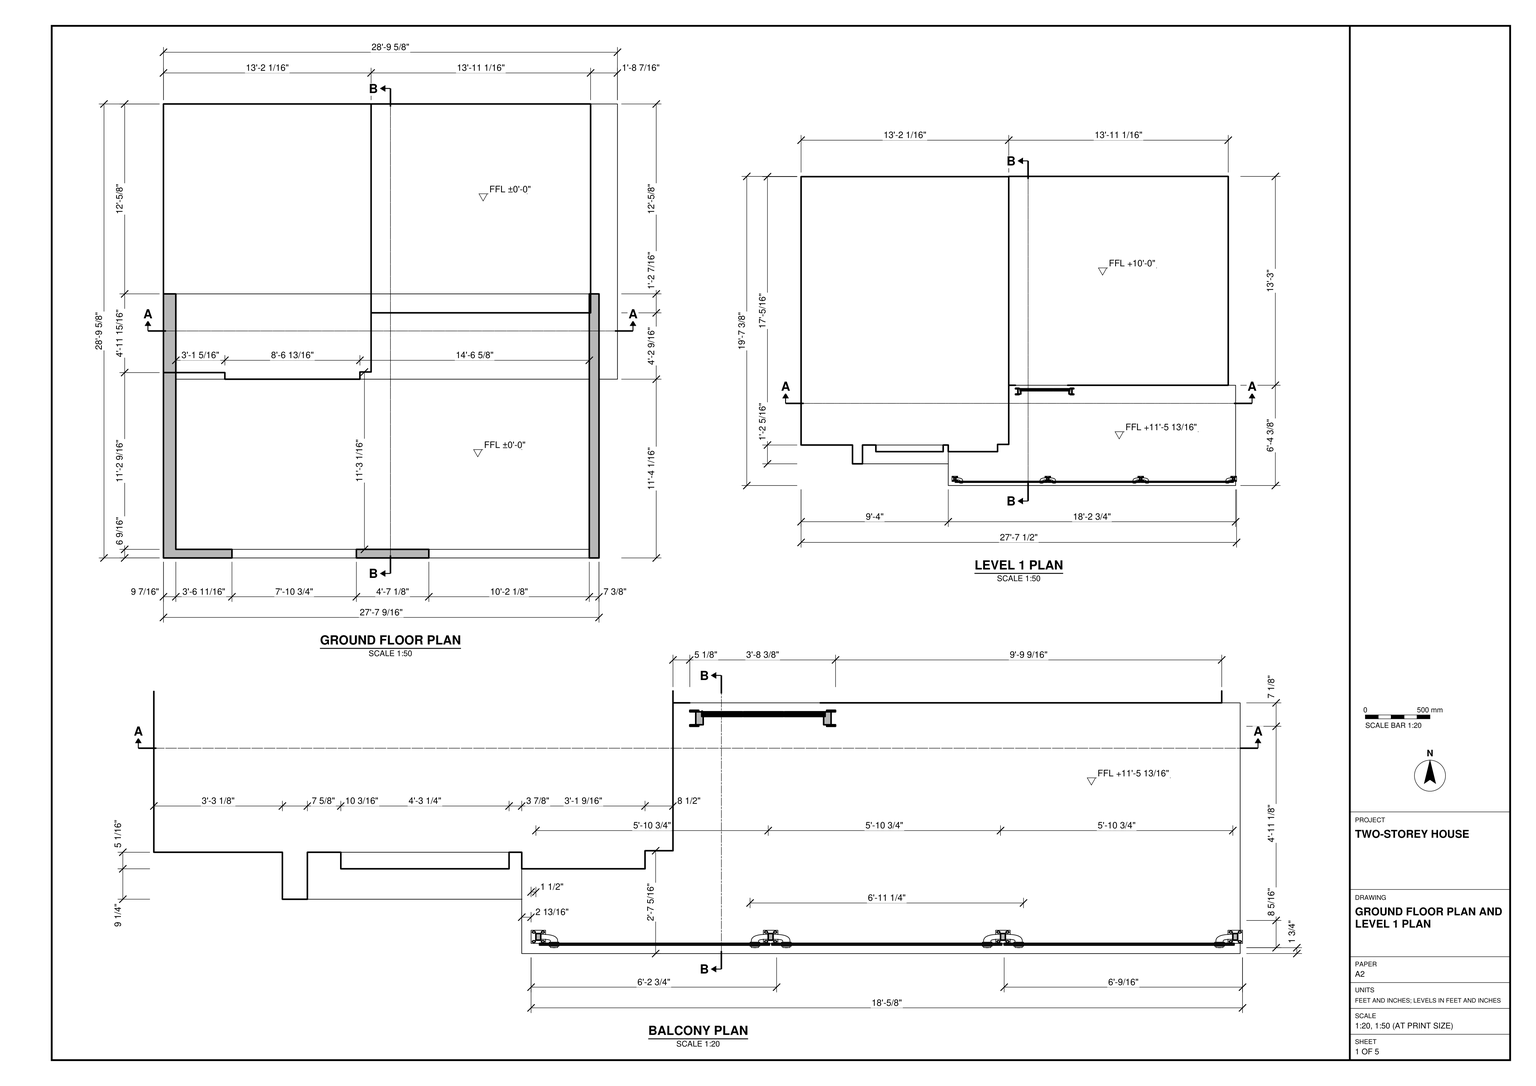
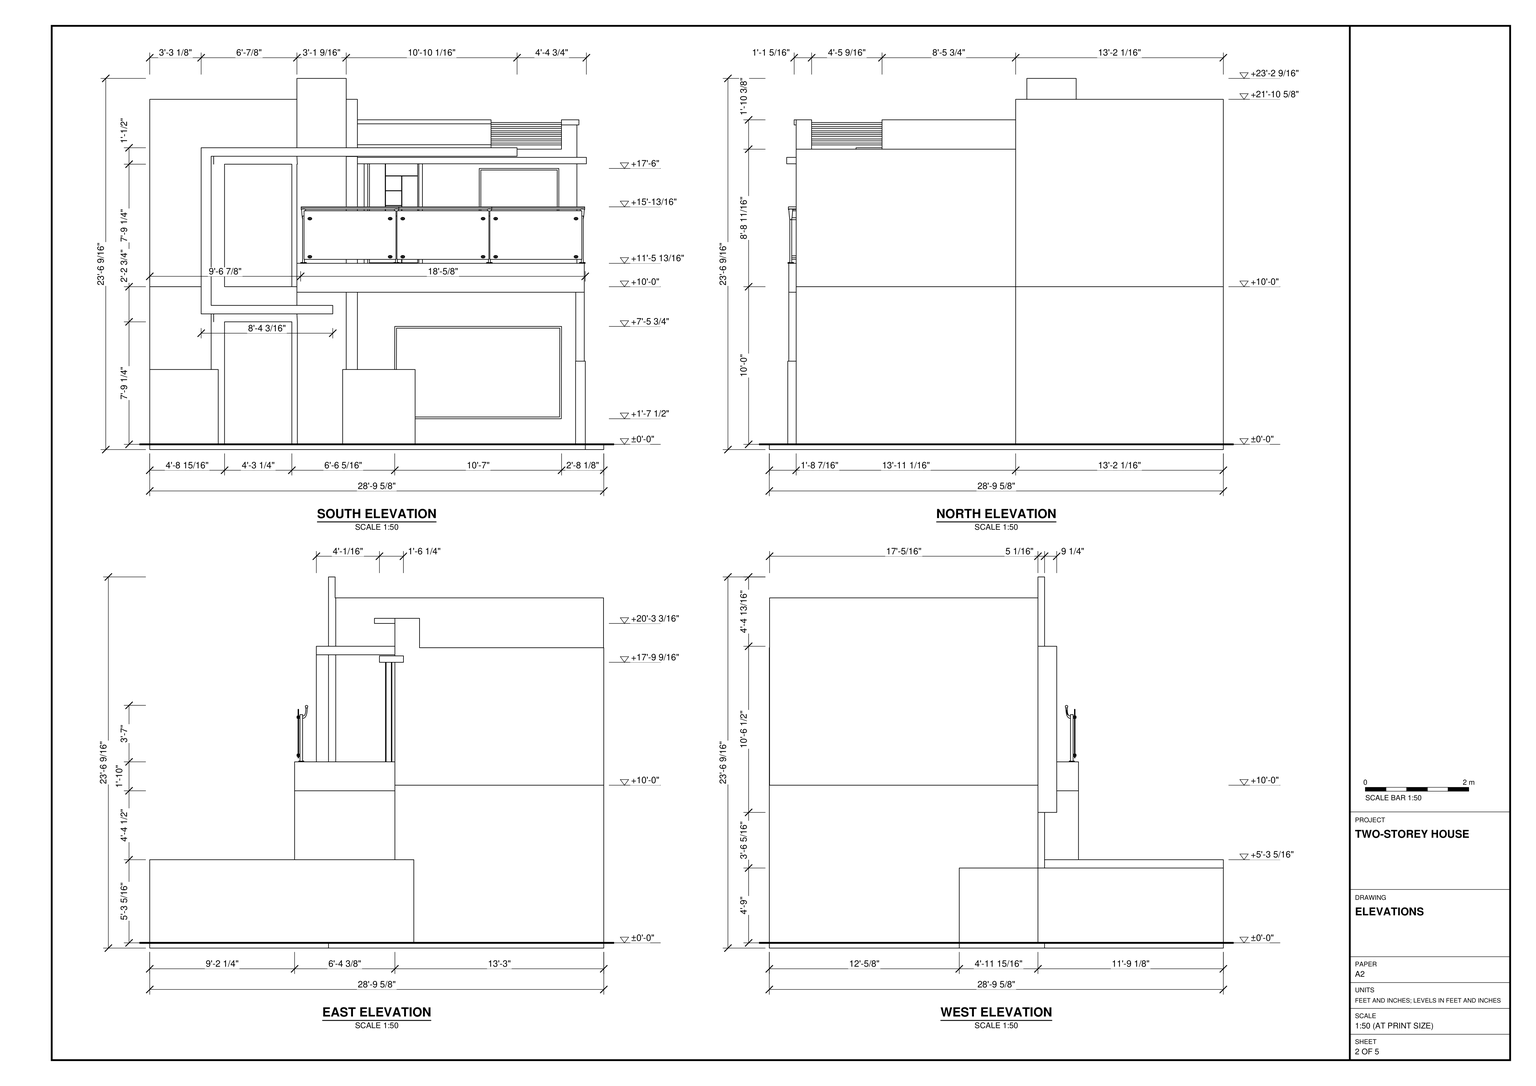
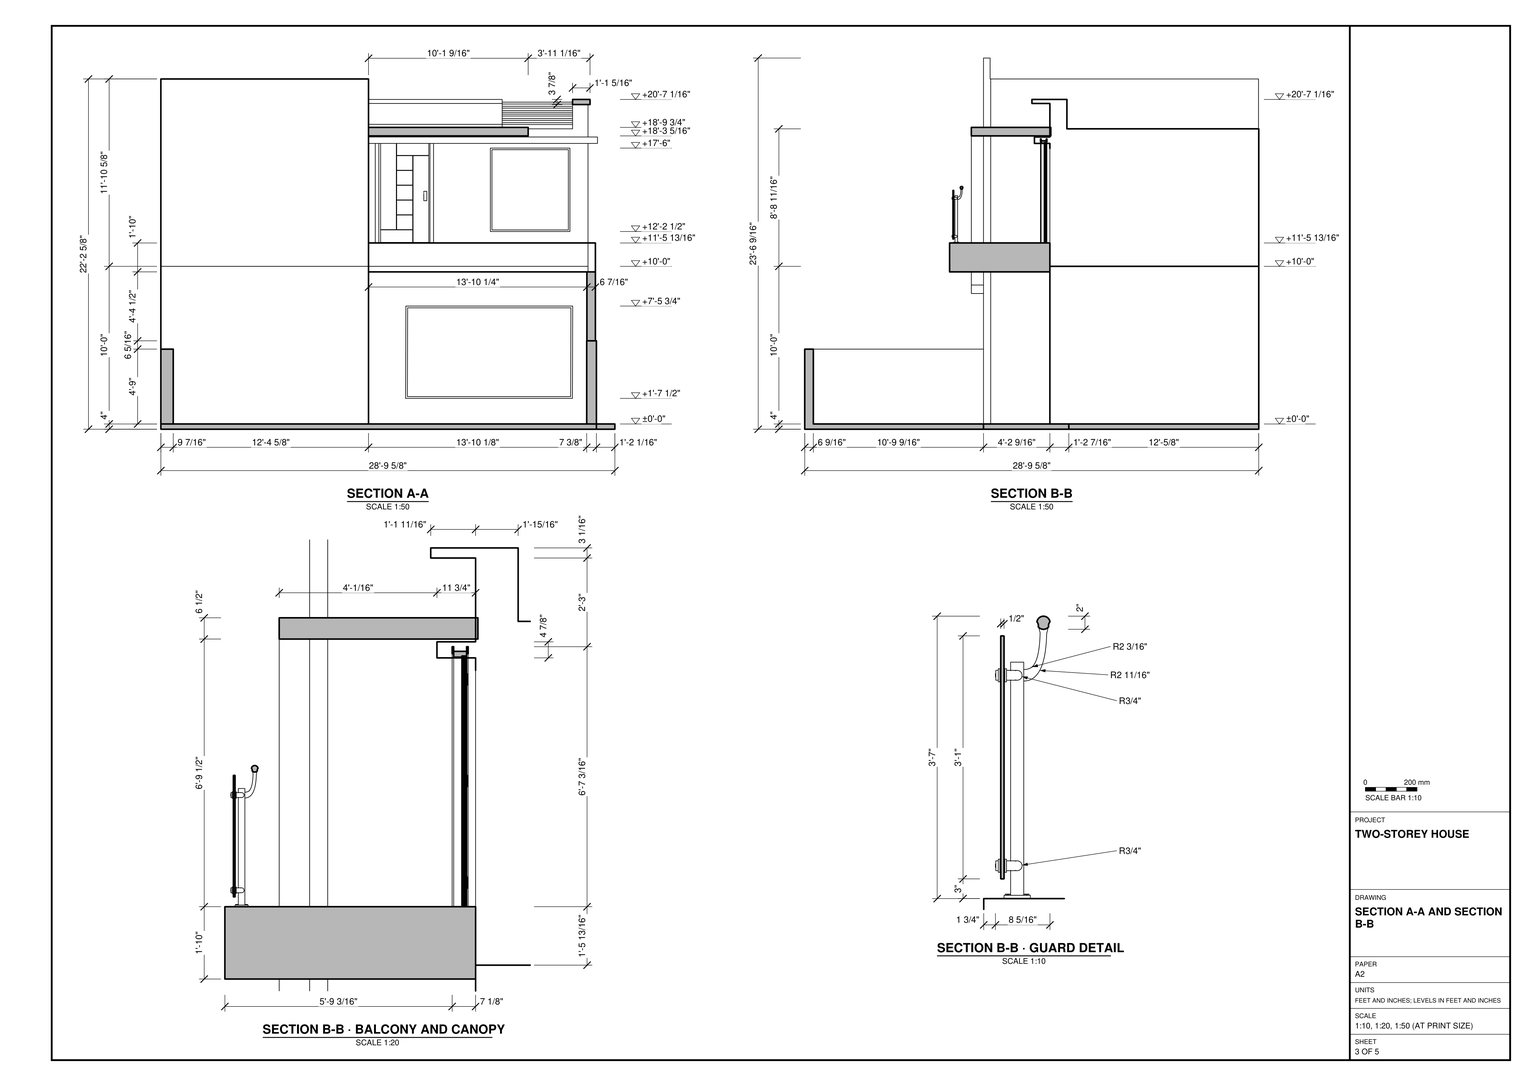
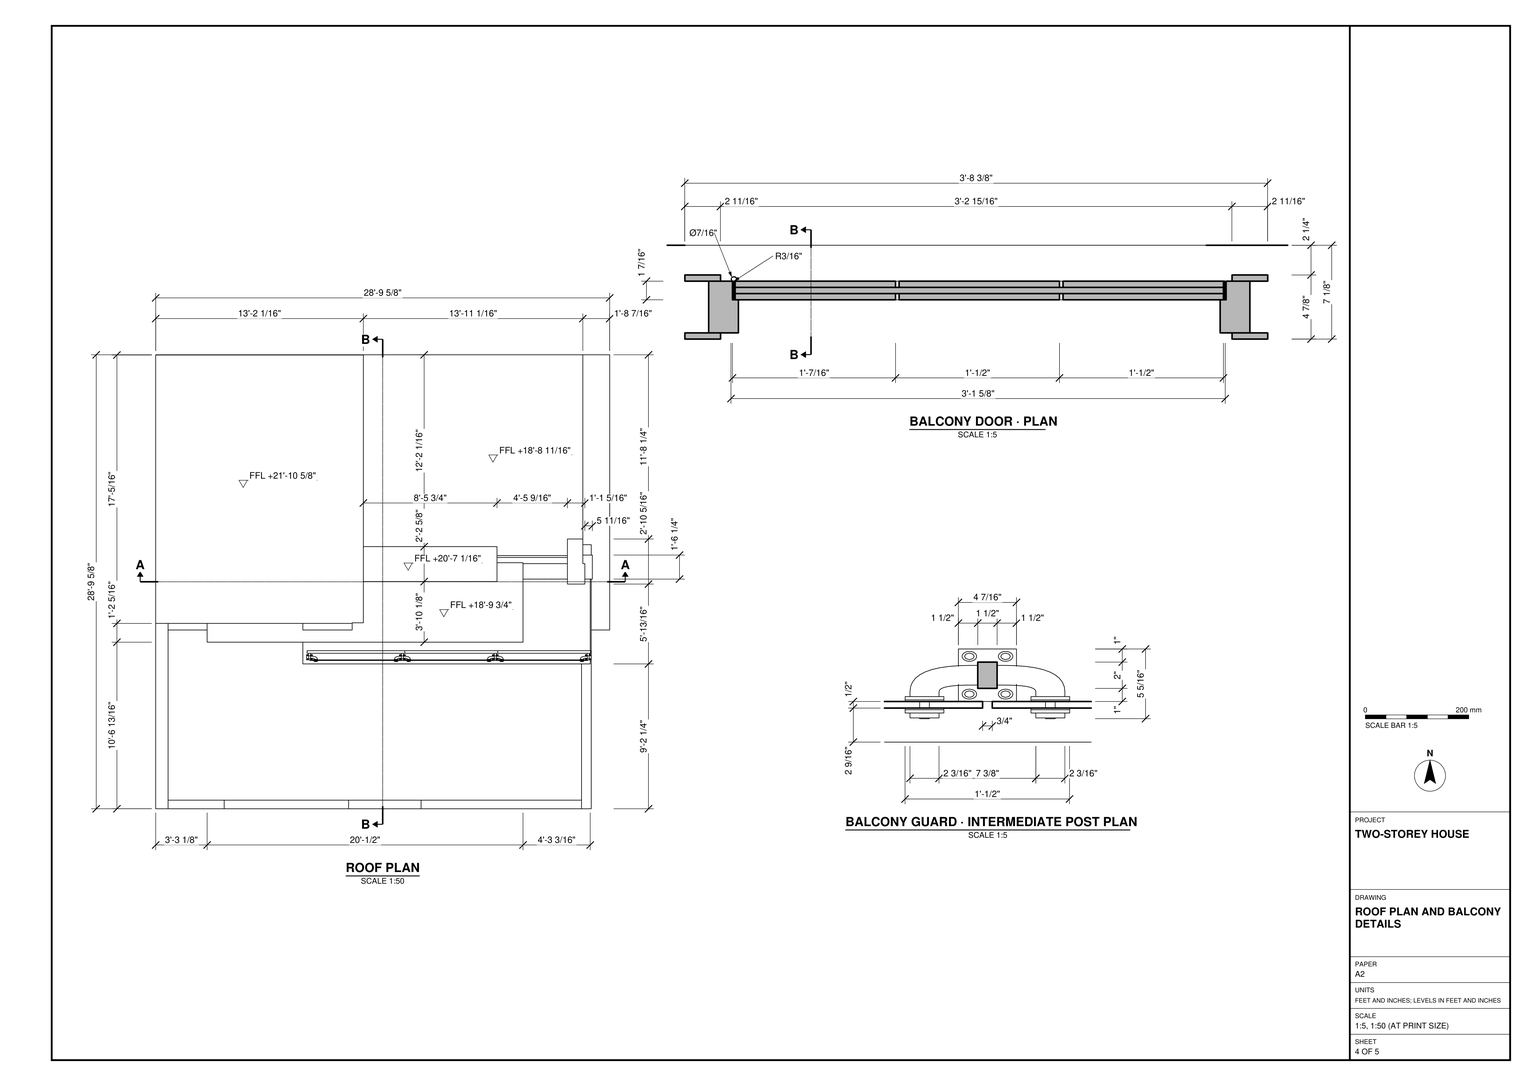
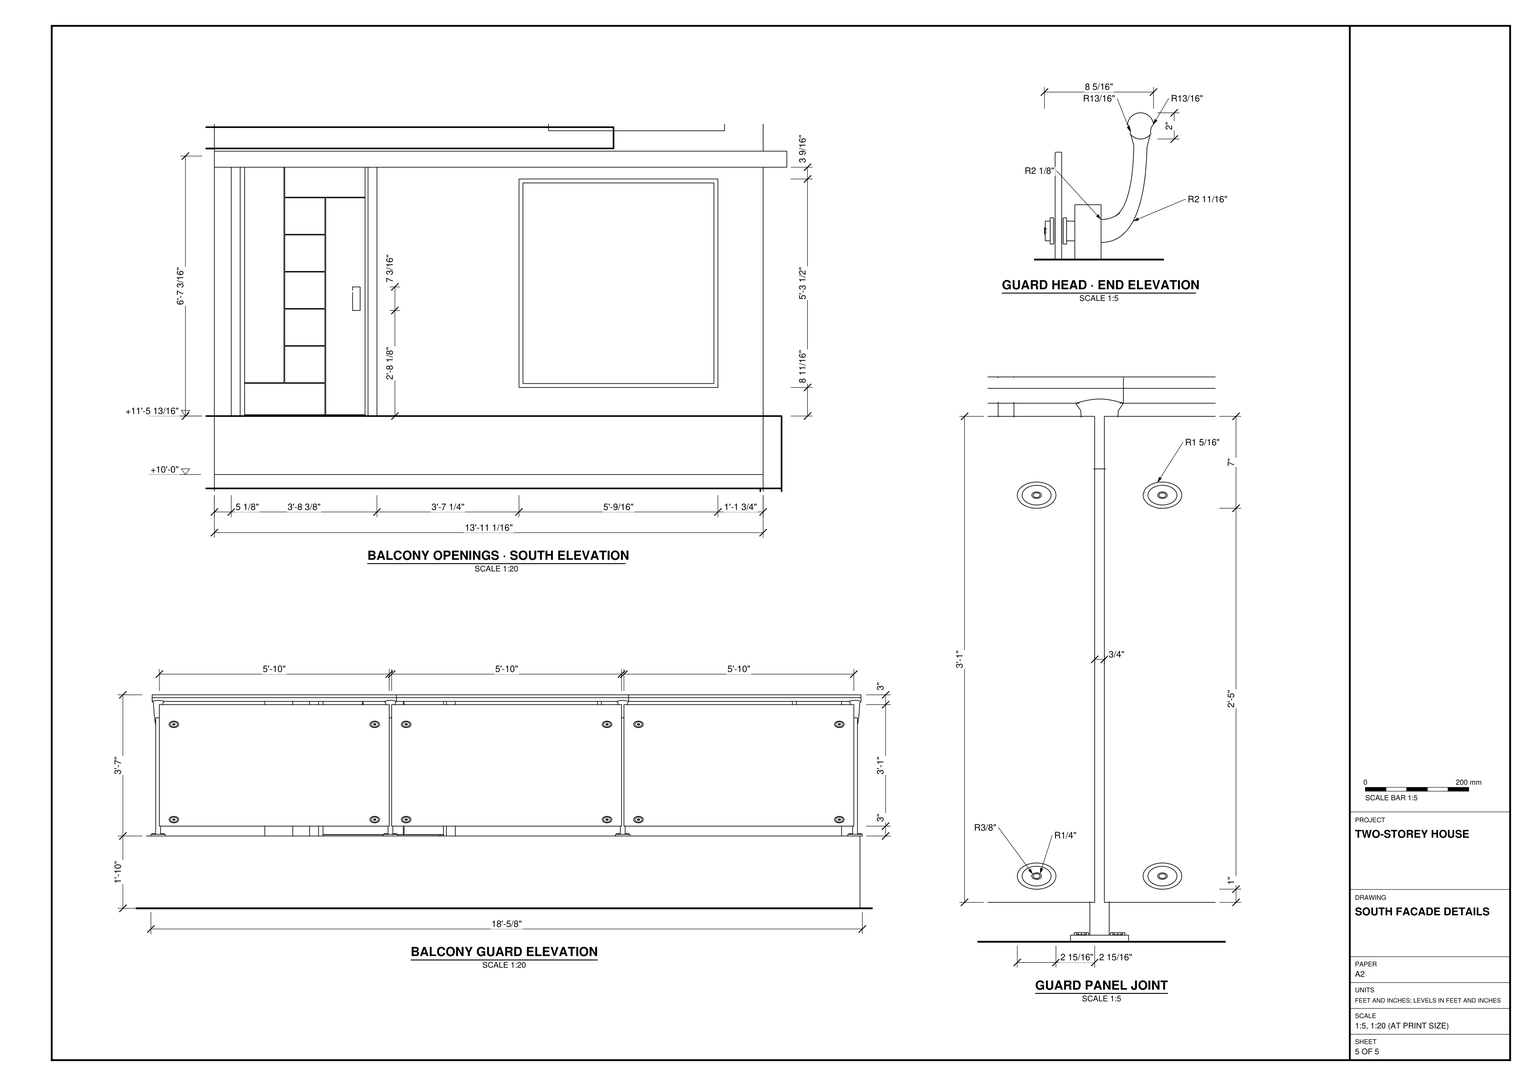
Build the two-storey house in SketchUp from task_files/diagram_01.pdf. Work in feet and inches. The model measures 28'-9 5/8" east to west, 28'-9 5/8" north to south and 23'-6 9/16" overall in height. Set the ground floor at ±0'-0" and the upper floor at +10'-0". The balcony surface is higher than the upper floor, at +11'-5 13/16".

Start with the square base slab and use the plans to position the taller west block and the recessed east bay. Model the walls at their drawn thicknesses, including the low side walls and the short wall sections that leave gaps along the south edge. Follow the elevations for the flat roofs, stepped parapets and projecting frame on the south face. Set the broad ground-floor window below the balcony and place the upper door and window behind it. Use the balcony plan for the slab outline and the sections for the canopy projection and guard construction. Show the glass panels, posts, panel fixings and offset handrail.

Keep walls, slabs and roofs in separate groups or components, and do the same for each furniture or joinery piece shown. Use components for repeated parts such as railing posts. Any decor or loose items shown may be suitable library components. Save one SketchUp model as output_files/two_storey_house_with_a_raised_front_balcony.skp.

# SketchUp Ruby script. Lengths in inches.
U = 1.inch
M = Sketchup.active_model
def pt(a) = Geom::Point3d.new(a.map { |v| v * U })
def face(e, loops, mat)
  f = e.add_face(loops[0].map { |a| pt(a) })
  loops[1..].each { |l| e.add_face(l.map { |a| pt(a) }).erase! }
  f.material = f.back_material = mat if mat
  f
end
# faces: each face lists its corners as indices into pts; further lists are holes
def faces(e, pts, list, mat = nil) = list.each { |f| face(e, (f[0].is_a?(Array) ? f : [f]).map { |l| l.map { |i| pts[i] } }, mat) }
# xy, xz, yz: faces in a plane at the given z, y or x. An outline is a flat list of corners, or four numbers for a rectangle; further outlines are holes
def ring(l) = l.size == 4 ? [[l[0], l[1]], [l[2], l[1]], [l[2], l[3]], [l[0], l[3]]] : l.each_slice(2).to_a
def flat(e, list, mat, &to3) = list.each { |f| face(e, (f[0].is_a?(Array) ? f : [f]).map { |l| ring(l).map { |u, v| to3.(u, v) } }, mat) }
def xy(e, z, list, mat = nil) = flat(e, list, mat) { |x, y| [x, y, z] }
def xz(e, y, list, mat = nil) = flat(e, list, mat) { |x, z| [x, y, z] }
def yz(e, x, list, mat = nil) = flat(e, list, mat) { |y, z| [x, y, z] }
def lines(e, pts, list) = list.each { |a, b| e.add_line(pt(pts[a]), pt(pts[b])) }
# prism: a flat outline (further loops are holes) pulled along v
def prism(e, loops, v, mat = nil)
  f = face(e, loops, mat); d = Geom::Vector3d.new(v.map { |x| x * U })
  f.pushpull(f.normal.samedirection?(d) ? d.length : -d.length)
end
def box(e, o, s, mat = nil) = prism(e, [[o, [o[0] + s[0], o[1], o[2]], [o[0] + s[0], o[1] + s[1], o[2]], [o[0], o[1] + s[1], o[2]]]], [0, 0, s[2]], mat)
def at(x, y, z, deg = 0) = Geom::Transformation.translation(pt([x, y, z])) * Geom::Transformation.rotation(ORIGIN, Z_AXIS, deg.degrees)
def axes(o, x, y, z) = Geom::Transformation.new([*x, 0, *y, 0, *z, 0, *pt(o).to_a, 1])
def part(name) = M.definitions.add(name)
# library, detail: a bought-in or finely detailed component or shape, given as its bounding box
def library(name, o, s) = part(name).tap { |d| box(d.entities, o, s) }
def detail(e, o, s) = box(e.add_group.entities, o, s)
def put(e, d, t, mat = nil) = e.add_instance(d, t).tap { |i| i.material = mat if mat }
def group(e, t, mat = nil) = e.add_group.tap { |g| g.transformation = t; g.material = mat if mat }.entities
root = M.entities
M.materials.add("B07_Copper_Blaze").color = [153, 35, 0]
M.materials.add("B08_Burnt_Sienna").color = [102, 25, 0]
M.materials.add("C02_Golden_Beige").color = [255, 205, 155]
M.materials.add("C07_Caramel_Shine").color = [153, 76, 0]
M.materials.add("D04_Dandelion_Burst").color = [255, 204, 50]
M.materials.add("E06_Meadow_Fresh").color = [204, 204, 0]
M.materials.add("Generic").color = [255, 255, 255]
M.materials.add("Glass_Basic_01").color = [161, 173, 186]
M.materials["Glass_Basic_01"].alpha = 0.25
M.materials.add("Glass_Safety_01").color = [204, 235, 244]
M.materials["Glass_Safety_01"].alpha = 0.25
M.materials.add("Glass_Safety_1").color = [204, 235, 244]
M.materials["Glass_Safety_1"].alpha = 0.25
M.materials.add("Grid_60x30_2K").color = [253, 253, 253]
M.materials.add("Marble_01_1K").color = [230, 221, 211]
M.materials.add("Marble_06_1K").color = [165, 150, 147]
M.materials.add("Plank_Floor_1K").color = [252, 252, 252]
c1 = library("CP-00619 (91x220)",[-1.57,-0.47,0],[38.58,7.14,88.1875])
c2 = library("GlassRailing",[-49.5,-2.3125,0],[147,8.3,43])
box(root,[324.32,110.28,67.3],[6.47,76.34,52.47])
xy(root,0,[[324.21,0,325.17,186.625]])
xy(root,124,[[158.08,186.625,325.17,345.64]])
xy(root,217.57,[[158.08,174.86,158.08,186.625,325.17,186.625,325.17,193.14,332.39,193.14,332.39,174.86]],"D04_Dandelion_Burst")
xy(root,222.47,[[158.08,174.86,332.39,174.86,332.39,193.14,325.17,193.14,325.17,186.625,158.08,186.625]],"D04_Dandelion_Burst")
xy(root,228.68,[[259.82,186.625,313.41,186.625,313.41,205.38,325.17,205.38,325.17,345.64,158.08,345.64,158.08,199.59,259.82,199.59]])
xy(root,235.04,[[259.82,191.32,313.41,192.75]])
xy(root,236.44,[[259.82,191.32,313.41,192.75]])
xy(root,238.48,[[259.63,191.32,313.41,192.75]])
xy(root,239.88,[[259.63,191.32,313.41,192.75]])
xy(root,241.24,[[259.59,191.32,313.41,192.75]])
xy(root,242.64,[[259.59,191.32,313.41,192.75]])
xy(root,244.45,[[259.82,191.32,313.41,192.75]])
xy(root,245.85,[[259.82,191.32,313.41,192.75]])
xy(root,247.17,[[313.41,171.07,326.7,186.625]])
xy(root,247.59,[[259.34,191.32,313.41,192.75]])
xy(root,247.98,[[158.08,172.97,259.82,186.625]],"Plank_Floor_1K")
xy(root,248.99,[[259.34,191.32,313.41,192.75]])
xy(root,251.05,[[313.41,171.07,326.7,171.07,326.7,186.625,325.17,186.625,325.17,205.38,313.41,205.38],[158.08,172.97,259.82,199.59]])
xz(root,171.07,[[313.41,247.17,326.7,251.05]])
xz(root,172.97,[[158.08,247.98,259.82,251.05]],"C02_Golden_Beige")
xz(root,174.86,[[158.08,217.57,332.39,222.47]],"D04_Dandelion_Burst")
xz(root,186.625,[[[158.08,124,325.17,217.57],[250.84,150.5,311.4,214],[163.21,141.8,202.89,213.79]],[158.08,222.47,325.17,222.47,325.17,247.17,313.41,247.17,313.41,228.68,259.82,228.68,259.82,232.1,158.08,232.1],[325.17,247.17,326.7,251.05]])
xz(root,186.625,[[[250.84,150.5,311.4,214],[252.04,151.71,310.2,212.8]]],"E06_Meadow_Fresh")
xz(root,186.625,[[252.04,151.71,310.2,212.8]],"Glass_Safety_1")
xz(root,186.625,[[158.08,232.1,259.82,247.98]],"Plank_Floor_1K")
xz(root,191.32,[[259.82,231.95,313.41,233.35],[259.82,235.04,313.41,236.44],[259.63,238.48,313.41,239.88],[259.59,241.24,313.41,242.64],[259.82,244.45,313.41,245.85],
  [259.34,247.59,313.41,248.99]])
xz(root,192.75,[[259.82,235.04,313.41,236.44],[259.63,238.48,313.41,239.88],[259.59,241.24,313.41,242.64],[259.82,244.45,313.41,245.85],[259.34,247.59,313.41,248.99]])
xz(root,193.14,[[325.17,217.57,332.39,222.47]])
xz(root,199.59,[[158.08,228.68,259.82,251.05]])
xz(root,205.38,[[313.41,228.68,325.17,251.05]])
xz(root,345.64,[[158.08,124,325.17,228.68]])
yz(root,158.08,[[186.625,124,186.625,217.57,174.86,217.57,174.86,222.47,186.625,222.47,186.625,247.98,172.97,247.98,172.97,251.05,199.59,251.05,199.59,228.68,345.64,228.68,345.64,124]])
yz(root,259.34,[[191.32,247.59,192.75,248.99]])
yz(root,259.59,[[191.32,241.24,192.75,242.64]])
yz(root,259.63,[[191.32,238.48,192.75,239.88]])
yz(root,259.82,[[[186.625,228.68,199.59,228.68,199.59,251.05,172.97,251.05,172.97,247.98,186.625,247.98],[191.32,235.04,192.75,236.44],[191.32,244.45,192.75,245.85]]])
yz(root,313.41,[[[186.625,228.68,186.625,247.17,171.07,247.17,171.07,251.05,205.38,251.05,205.38,228.68],[191.32,247.59,192.75,248.99],[191.32,244.45,192.75,245.85],[191.32,241.24,192.75,242.64],[191.32,238.48,192.75,239.88],[191.32,235.04,192.75,236.44]]])
yz(root,325.17,[[186.625,124,345.64,124,345.64,228.68,205.38,228.68,205.38,251.05,186.625,251.05,186.625,222.47,193.14,222.47,193.14,217.57,186.625,217.57]])
yz(root,326.7,[[171.07,247.17,186.625,251.05]])
yz(root,332.39,[[174.86,217.57,193.14,222.47]],"D04_Dandelion_Burst")
p = [[313.41,192.75,233.35],[259.82,192.75,233.35]]
lines(root,p,[[0,1]])
put(root,c1,axes([165.02,179.96,141.8],[1.15,0,0],[0,1,0],[0,0,0.89784]))
put(root,c2,axes([187.8125,114.37,141.8],[1.47371,0,0],[0,1,0],[0,0,1]))
g1 = group(root,at(24.45,136.09,0))
box(g1,[-24.45,0,0],[345.62,209.54,4])
g2 = group(root,at(0,126.82,4))
xy(g2,0,[[46.75,9.27,46.75,14.31,0,14.31,0,218.8125,158.08,218.8125,158.08,14.77,149.57,14.77,149.57,9.27],[158.08,59.81,325.17,218.8125]])
xy(g2,99.3,[[46.75,0,48.67,9.27],[48.67,0,49.05,9.27],[49.05,0,139.32,9.27]])
xy(g2,99.3,[[39.14,0,46.75,14.31]],"Plank_Floor_1K")
xy(g2,105.78,[[46.75,0,139.32,0,139.32,9.27,112.03,9.27,112.03,14.31,46.75,14.31]])
xy(g2,115.77,[[112.03,-16.54,112.03,9.27,149.57,9.27,149.57,14.77,158.08,14.77,158.08,59.81,330.79,59.81,330.79,-16.54]],"Marble_06_1K")
xy(g2,120,[[56.9375,9.27,108.17,14.31],[158.08,59.81,325.17,218.8125],[0,218.62,158.08,218.8125]])
xy(g2,137.8,[[112.03,-16.54,330.79,-16.54,330.79,59.81,158.08,59.81,158.08,14.77,149.57,14.77,149.57,9.27,112.03,9.27]],"Generic")
xy(g2,213.26,[[56.9375,9.27,108.17,14.31],[112.03,9.27,112.36,14.31]],"C07_Caramel_Shine")
xy(g2,219.3,[[46.75,0,48.67,14.31],[48.67,0,49.05,14.31],[49.05,0,49.05,14.31,112.03,14.31,112.03,9.27,149.57,9.27,149.57,14.77,158.08,14.77,158.08,60.51,279.62,60.51,279.62,0]])
xy(g2,225.78,[[39.14,0,279.62,0,279.62,60.51,158.08,60.51,158.08,14.77,149.57,14.77,149.57,9.27,112.03,9.27,112.03,14.31,39.14,14.31]],"Plank_Floor_1K")
xy(g2,262.64,[[0,14.31,149.57,14.31,149.57,14.77,158.08,14.77,158.08,218.62,0,218.62]])
xy(g2,278.58,[[112.03,9.27,149.57,14.31]])
xz(g2,-16.54,[[112.03,115.77,330.79,137.8]],"Generic")
xz(g2,0,[[39.14,99.3,139.32,99.3,139.32,105.78,46.75,105.78,46.75,219.3,279.62,219.3,279.62,225.78,39.14,225.78]],"Plank_Floor_1K")
xz(g2,9.27,[[46.75,0,56.9375,0,56.9375,93.26,108.17,93.26,108.17,0,112.36,0,112.36,93.26,112.03,99.3,46.75,99.3]],"B07_Copper_Blaze")
xz(g2,9.27,[[56.9375,0,108.17,93.26],[56.9375,120,108.17,213.26]],"Glass_Basic_01")
xz(g2,9.27,[[112.36,0,149.57,0,149.57,115.77,112.03,115.77,112.03,105.78,139.32,105.78,139.32,99.3,112.03,99.3,112.36,93.26],[112.03,137.8,149.57,137.8,149.57,219.3,112.03,219.3,112.36,213.26,112.03,213.26],[112.03,225.78,149.57,278.58]],"Marble_06_1K")
xz(g2,14.31,[[112.03,262.64,149.57,278.58]])
xz(g2,14.31,[[46.75,105.78,112.03,105.78,112.03,120,56.9375,120,56.9375,213.26,108.17,213.26,108.17,120,112.03,120,112.03,213.26,112.36,213.26,112.03,219.3,46.75,219.3]],"B07_Copper_Blaze")
xz(g2,14.31,[[0,0,46.75,0,46.75,99.3,39.14,99.3,39.14,120,0,120],[0,120,39.14,120,39.14,225.78,112.03,225.78,112.03,262.64,0,262.64]],"Plank_Floor_1K")
xz(g2,14.77,[[149.57,0,158.08,115.77],[149.57,137.8,158.08,219.12]],"B07_Copper_Blaze")
xz(g2,14.77,[[149.57,115.77,158.08,137.8]],"Generic")
xz(g2,14.77,[[149.57,219.12,158.08,219.3],[149.57,219.3,158.08,225.78],[149.57,225.78,158.08,262.64]],"Grid_60x30_2K")
xz(g2,59.81,[[[158.08,0,325.17,115.77],[186.32,19.49,186.51,89.76,313.49,89.76,313.31,19.49]],[158.08,115.77,325.17,120]])
xz(g2,59.81,[[[186.32,19.49,313.31,19.49,313.49,89.76,186.51,89.76],[187.67,20.83,187.85,88.42,312.15,88.42,311.96,20.83]]],"B08_Burnt_Sienna")
xz(g2,59.81,[[325.17,115.77,325.17,120,158.08,120,158.08,137.8,330.79,137.8,330.79,115.77]],"Generic")
xz(g2,59.81,[[187.67,20.83,311.96,20.83,312.15,88.42,187.85,88.42]],"Glass_Safety_01")
xz(g2,60.51,[[158.08,219.3,279.62,225.78]])
xz(g2,218.62,[[0,120,158.08,262.64]])
xz(g2,218.8125,[[0,0,158.08,120],[158.08,0,325.17,120]])
yz(g2,0,[[14.31,0,218.8125,120],[14.31,120,218.62,262.64]])
yz(g2,39.14,[[0,99.3,14.31,225.78]],"Plank_Floor_1K")
yz(g2,46.75,[[9.27,0,14.31,99.3],[0,105.78,14.31,120],[0,120,14.31,219.3]],"Plank_Floor_1K")
yz(g2,56.9375,[[9.27,120,14.31,213.26]],"C07_Caramel_Shine")
yz(g2,108.17,[[9.27,120,14.31,213.26]],"C07_Caramel_Shine")
yz(g2,112.03,[[9.27,225.78,14.31,278.58]])
yz(g2,112.03,[[9.27,105.78,9.27,115.77,-16.54,115.77,-16.54,137.8,9.27,137.8,9.27,213.26,14.31,213.26,14.31,105.78]],"Generic")
yz(g2,139.32,[[0,99.3,9.27,105.78]])
yz(g2,149.57,[[9.27,0,14.77,115.77],[9.27,137.8,14.77,219.3],[9.27,225.78,14.77,225.78,14.77,262.64,14.31,262.64,14.31,278.58,9.27,278.58]],"Generic")
yz(g2,158.08,[[14.77,0,59.81,115.77],[59.81,0,218.8125,120],[59.81,120,218.62,120,218.62,262.64,14.77,262.64,14.77,225.78,60.51,225.78,60.51,219.3,14.77,219.3,14.77,137.8,59.81,137.8],[14.77,219.3,60.51,225.78]])
yz(g2,158.08,[[14.77,115.77,59.81,120],[14.77,120,59.81,137.8]],"Generic")
yz(g2,279.62,[[0,219.3,60.51,225.78]])
yz(g2,325.17,[[59.81,0,218.8125,120]])
yz(g2,330.79,[[-16.54,115.77,59.81,137.8]],"Generic")
p = [[112.36,9.27,213.26],[112.03,9.27,219.3],[112.03,14.31,219.3],[112.36,14.31,213.26],[48.67,14.31,213.26],[48.67,14.31,219.3],
  [48.67,9.27,93.26],[48.67,9.27,99.3]]
faces(g2,p,[[0,1,2,3]],"C07_Caramel_Shine")
lines(g2,p,[[4,5],[6,7]])
g3 = group(root,at(0,0,0),"Marble_06_1K")
xy(g3,0,[[0,0,331.57,201.04]])
xy(g3,4,[[52.14,0,146.87,6.55],[202.02,0,324.17,6.55]])
xy(g3,4,[[9.43,6.55,324.17,201.04]],"Marble_01_1K")
xy(g3,60.97,[[0,0,9.43,201.04],[9.43,0,52.14,6.55],[146.87,0,202.02,6.55]])
xy(g3,67.3,[[324.17,0,331.57,201.04]])
xz(g3,0,[[0,0,331.57,0,331.57,67.3,324.17,67.3,324.17,4,202.02,4,202.02,60.97,146.87,60.97,146.87,4,52.14,4,52.14,60.97,0,60.97]])
xz(g3,6.55,[[9.43,4,52.14,60.97],[146.87,4,202.02,60.97]])
xz(g3,201.04,[[0,0,0,60.97,9.43,60.97,9.43,4,324.17,4,324.17,67.3,331.57,67.3,331.57,0]])
yz(g3,0,[[0,0,201.04,60.97]])
yz(g3,9.43,[[6.55,4,201.04,60.97]])
yz(g3,52.14,[[0,4,6.55,60.97]])
yz(g3,146.87,[[0,4,6.55,60.97]])
yz(g3,202.02,[[0,4,6.55,60.97]])
yz(g3,324.17,[[0,4,201.04,67.3]])
yz(g3,331.57,[[0,0,201.04,67.3]])
